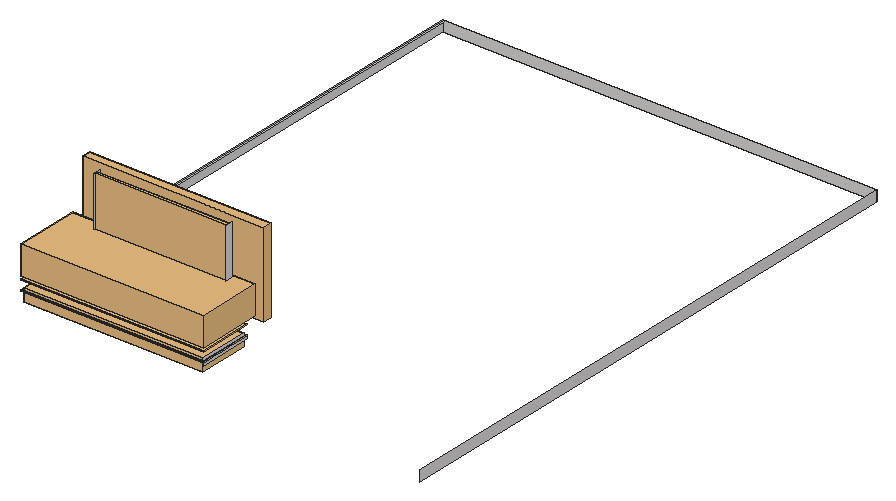
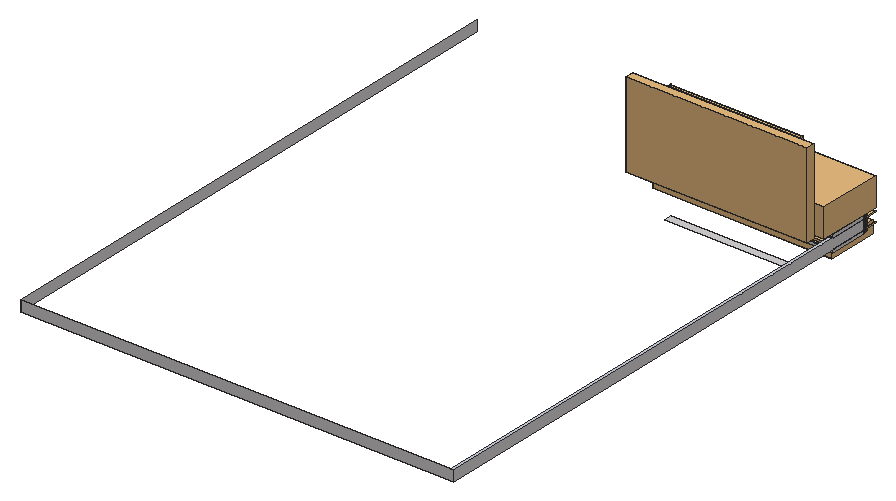
# SketchUp Ruby script. Lengths in inches.
U = 1.inch
M = Sketchup.active_model
def pt(a) = Geom::Point3d.new(a.map { |v| v * U })
def face(e, loops, mat)
  f = e.add_face(loops[0].map { |a| pt(a) })
  loops[1..].each { |l| e.add_face(l.map { |a| pt(a) }).erase! }
  f.material = f.back_material = mat if mat
  f
end
# faces: each face lists its corners as indices into pts; further lists are holes
def faces(e, pts, list, mat = nil) = list.each { |f| face(e, (f[0].is_a?(Array) ? f : [f]).map { |l| l.map { |i| pts[i] } }, mat) }
# xy, xz, yz: faces in a plane at the given z, y or x. An outline is a flat list of corners, or four numbers for a rectangle; further outlines are holes
def ring(l) = l.size == 4 ? [[l[0], l[1]], [l[2], l[1]], [l[2], l[3]], [l[0], l[3]]] : l.each_slice(2).to_a
def flat(e, list, mat, &to3) = list.each { |f| face(e, (f[0].is_a?(Array) ? f : [f]).map { |l| ring(l).map { |u, v| to3.(u, v) } }, mat) }
def xy(e, z, list, mat = nil) = flat(e, list, mat) { |x, y| [x, y, z] }
def xz(e, y, list, mat = nil) = flat(e, list, mat) { |x, z| [x, y, z] }
def yz(e, x, list, mat = nil) = flat(e, list, mat) { |y, z| [x, y, z] }
def lines(e, pts, list) = list.each { |a, b| e.add_line(pt(pts[a]), pt(pts[b])) }
# prism: a flat outline (further loops are holes) pulled along v
def prism(e, loops, v, mat = nil)
  f = face(e, loops, mat); d = Geom::Vector3d.new(v.map { |x| x * U })
  f.pushpull(f.normal.samedirection?(d) ? d.length : -d.length)
end
def box(e, o, s, mat = nil) = prism(e, [[o, [o[0] + s[0], o[1], o[2]], [o[0] + s[0], o[1] + s[1], o[2]], [o[0], o[1] + s[1], o[2]]]], [0, 0, s[2]], mat)
def at(x, y, z, deg = 0) = Geom::Transformation.translation(pt([x, y, z])) * Geom::Transformation.rotation(ORIGIN, Z_AXIS, deg.degrees)
def axes(o, x, y, z) = Geom::Transformation.new([*x, 0, *y, 0, *z, 0, *pt(o).to_a, 1])
def part(name) = M.definitions.add(name)
# library, detail: a bought-in or finely detailed component or shape, given as its bounding box
def library(name, o, s) = part(name).tap { |d| box(d.entities, o, s) }
def detail(e, o, s) = box(e.add_group.entities, o, s)
def put(e, d, t, mat = nil) = e.add_instance(d, t).tap { |i| i.material = mat if mat }
def group(e, t, mat = nil) = e.add_group.tap { |g| g.transformation = t; g.material = mat if mat }.entities
root = M.entities
M.materials.add("Outer Light - 1").color = [251, 216, 141]
M.materials.add("T METAL").color = [42, 41, 39]
M.materials.add("[Marble Carrara Floor Tile]").color = [204, 208, 219]
M.materials.add("[Quartz Light Brown]").color = [215, 212, 212]
c1 = library("Group\#43",[-0.5,-0.5,0],[204,61,1])
c2 = library("Group\#47",[0,0,-15.9],[195,66,15.9])
c3 = library("Group\#42",[-0.5,-0.5,0],[204,61,1])
c4 = library("Group\#21",[0,0,0],[201,72,32])
c5 = library("Glass Door Sliding Door 4 Panel on 2 Tracks _ Model by Pooh",[0,0,0],[157.59,4.01,102.67])
c6 = library("Garniza_zaclona",[1.52,0,0],[127.96,8.15,78.72])
xy(root,216,[[33,266,180,275]],"[Quartz Light Brown]")
xy(root,257.9,[[33,266,180,275]],"[Quartz Light Brown]")
xy(root,258,[[0,266,3,794]],"[Marble Carrara Floor Tile]")
xz(root,264,[[2,243,202,249]],"[Quartz Light Brown]")
xz(root,266,[[0,243,204,246],[0,246,0.5,247],[0,257,0.5,258],[0,258,3,261]],"[Quartz Light Brown]")
xz(root,794,[[0,246,483,258]],"[Quartz Light Brown]")
yz(root,0,[[222.76,243,223,246],[223,243,266,246],[266,246,266,247,223,247,223,257,266,257,266,258,794,258,794,246],[222.76,247,223,257],[222.76,258,223,261],
  [223,258,266,261]],"[Quartz Light Brown]")
yz(root,0.01,[[222.29,243,222.53,246],[222.29,247,222.53,257],[222.29,258,222.53,261]],"[Quartz Light Brown]")
yz(root,0.5,[[222.77,246,223,247],[223,246,266,247],[222.77,257,223,258],[223,257,266,258]],"[Quartz Light Brown]")
yz(root,0.51,[[222.3125,246,222.54,247],[222.3125,257,222.54,258]],"[Quartz Light Brown]")
yz(root,2,[[222.79,243,223,249],[223,243,264,249]],"[Quartz Light Brown]")
yz(root,2.01,[[222.37,243,222.58,249]],"[Quartz Light Brown]")
yz(root,3,[[222.8,258,223,261],[223,258,266,261]],"[Quartz Light Brown]")
yz(root,3.01,[[222.41,258,222.61,261]],"[Quartz Light Brown]")
yz(root,33,[[266,257.9,275,348]],"[Quartz Light Brown]")
yz(root,180,[[266,257.9,275,348]],"[Quartz Light Brown]")
yz(root,202,[[207,243,264,249]],"[Quartz Light Brown]")
yz(root,204,[[205,243,266,246]],"[Quartz Light Brown]")
yz(root,483,[[158,246,794,258]],"[Quartz Light Brown]")
p = [[1.2,216.55,246],[1.2,216.55,243],[1.28,216.33,243],[1.28,216.33,246],[3.38,216.49,249],[3.47,216.3,249],
  [3.47,216.3,243],[3.38,216.49,243],[1.11,216.77,246],[1.11,216.77,243],[3.3,216.68,249],[3.3,216.68,243],
  [3.22,216.88,249],[3.22,216.88,243],[1.03,216.99,246],[1.03,216.99,243],[3.14,217.07,249],[3.14,217.07,243],
  [0.96,217.21,246],[0.96,217.21,243],[3.0625,217.27,249],[3.0625,217.27,243],[0.88,217.4375,246],[0.88,217.4375,243],
  [2.99,217.46,249],[2.99,217.46,243],[0.81,217.66,246],[0.81,217.66,243],[2.92,217.66,249],[2.92,217.66,243],
  [0.74,217.89,246],[0.74,217.89,243],[2.85,217.86,249],[2.85,217.86,243],[0.68,218.11,246],[0.68,218.11,243],
  [2.78,218.06,249],[2.78,218.06,243],[0.61,218.34,246],[0.61,218.34,243],[2.72,218.26,249],[2.72,218.26,243],
  [0.55,218.57,246],[0.55,218.57,243],[2.66,218.46,249],[2.66,218.46,243],[2.6,218.66,249],[2.6,218.66,243],
  [0.5,218.8,246],[0.5,218.8,243],[2.55,218.86,249],[2.55,218.86,243],[0.44,219.03,246],[0.44,219.03,243],
  [2.49,219.0625,249],[2.49,219.0625,243],[0.39,219.26,246],[0.39,219.26,243],[2.44,219.26,249],[2.44,219.26,243],
  [0.35,219.49,246],[0.35,219.49,243],[2.39,219.47,249],[2.39,219.47,243],[0.3,219.72,246],[0.3,219.72,243],
  [2.35,219.67,249],[2.35,219.67,243],[0.26,219.95,246],[0.26,219.95,243],[2.31,219.88,249],[2.31,219.88,243],
  [2.27,220.08,249],[2.27,220.08,243],[0.22,220.18,246],[0.22,220.18,243],[2.23,220.29,249],[2.23,220.29,243],
  [0.1875,220.42,246],[0.1875,220.42,243],[2.2,220.5,249],[2.2,220.5,243],[0.15,220.65,246],[0.15,220.65,243],
  [2.17,220.7,249],[2.17,220.7,243],[0.125,220.88,246],[0.125,220.88,243],[2.14,220.91,249],[2.14,220.91,243],
  [0.1,221.12,246],[0.1,221.12,243],[2.11,221.12,249],[2.11,221.12,243],[0.08,221.35,246],[0.08,221.35,243],
  [2.09,221.33,249],[2.09,221.33,243],[2.07,221.54,249],[2.07,221.54,243],[0.06,221.59,246],[0.06,221.59,243],
  [2.05,221.74,249],[2.05,221.74,243],[0.04,221.82,246],[0.04,221.82,243],[2.03,221.95,249],[2.03,221.95,243],
  [0.02,222.06,246],[0.02,222.06,243],[2.02,222.16,249],[2.02,222.16,243],[0.01,222.29,246],[0.01,222.29,243],
  [2.01,222.37,249],[2.01,222.37,243],[0,222.76,246],[0,222.76,243],[0.01,222.53,243],[0.01,222.53,246],
  [2,222.79,249],[2.01,222.58,249],[2.01,222.58,243],[2,222.79,243],[1.75,216.52,247],[1.75,216.52,246],
  [1.83,216.3,246],[1.83,216.3,247],[1.66,216.73,247],[1.66,216.73,246],[1.58,216.94,247],[1.58,216.94,246],
  [1.5,217.16,247],[1.5,217.16,246],[1.43,217.375,247],[1.43,217.375,246],[1.36,217.59,247],[1.36,217.59,246],
  [1.29,217.8125,247],[1.29,217.8125,246],[1.22,218.03,247],[1.22,218.03,246],[1.16,218.25,247],[1.16,218.25,246],
  [1.1,218.47,247],[1.1,218.47,246],[1.04,218.69,247],[1.04,218.69,246],[0.98,218.91,247],[0.98,218.91,246],
  [0.93,219.14,247],[0.93,219.14,246],[0.88,219.36,247],[0.88,219.36,246],[0.84,219.59,247],[0.84,219.59,246],
  [0.79,219.8125,247],[0.79,219.8125,246],[0.75,220.04,247],[0.75,220.04,246],[0.72,220.26,247],[0.72,220.26,246],
  [0.68,220.49,247],[0.68,220.49,246],[0.65,220.72,247],[0.65,220.72,246],[0.62,220.94,247],[0.62,220.94,246],
  [0.6,221.17,247],[0.6,221.17,246],[0.57,221.4,247],[0.57,221.4,246],[0.55,221.625,247],[0.55,221.625,246],
  [0.54,221.86,247],[0.54,221.86,246],[0.52,222.08,247],[0.52,222.08,246],[0.51,222.3125,247],[0.51,222.3125,246],
  [0.5,222.77,247],[0.5,222.77,246],[0.51,222.54,246],[0.51,222.54,247],[1.2,216.55,257],[1.2,216.55,247],
  [1.28,216.33,247],[1.28,216.33,257],[1.11,216.77,257],[1.11,216.77,247],[1.03,216.99,257],[1.03,216.99,247],
  [0.96,217.21,257],[0.96,217.21,247],[0.88,217.4375,257],[0.88,217.4375,247],[0.81,217.66,257],[0.81,217.66,247],
  [0.74,217.89,257],[0.74,217.89,247],[0.68,218.11,257],[0.68,218.11,247],[0.61,218.34,257],[0.61,218.34,247],
  [0.55,218.57,257],[0.55,218.57,247],[0.5,218.8,257],[0.5,218.8,247],[0.44,219.03,257],[0.44,219.03,247],
  [0.39,219.26,257],[0.39,219.26,247],[0.35,219.49,257],[0.35,219.49,247],[0.3,219.72,257],[0.3,219.72,247],
  [0.26,219.95,257],[0.26,219.95,247],[0.22,220.18,257],[0.22,220.18,247],[0.1875,220.42,257],[0.1875,220.42,247],
  [0.15,220.65,257],[0.15,220.65,247],[0.125,220.88,257],[0.125,220.88,247],[0.1,221.12,257],[0.1,221.12,247],
  [0.08,221.35,257],[0.08,221.35,247],[0.06,221.59,257],[0.06,221.59,247],[0.04,221.82,257],[0.04,221.82,247],
  [0.02,222.06,257],[0.02,222.06,247],[0.01,222.29,257],[0.01,222.29,247],[0,222.76,257],[0,222.76,247],
  [0.01,222.53,247],[0.01,222.53,257],[1.75,216.52,258],[1.75,216.52,257],[1.83,216.3,257],[1.83,216.3,258],
  [1.66,216.73,258],[1.66,216.73,257],[1.58,216.94,258],[1.58,216.94,257],[1.5,217.16,258],[1.5,217.16,257],
  [1.43,217.375,258],[1.43,217.375,257],[1.36,217.59,258],[1.36,217.59,257],[1.29,217.8125,258],[1.29,217.8125,257],
  [1.22,218.03,258],[1.22,218.03,257],[1.16,218.25,258],[1.16,218.25,257],[1.1,218.47,258],[1.1,218.47,257],
  [1.04,218.69,258],[1.04,218.69,257],[0.98,218.91,258],[0.98,218.91,257],[0.93,219.14,258],[0.93,219.14,257],
  [0.88,219.36,258],[0.88,219.36,257],[0.84,219.59,258],[0.84,219.59,257],[0.79,219.8125,258],[0.79,219.8125,257],
  [0.75,220.04,258],[0.75,220.04,257],[0.72,220.26,258],[0.72,220.26,257],[0.68,220.49,258],[0.68,220.49,257],
  [0.65,220.72,258],[0.65,220.72,257],[0.62,220.94,258],[0.62,220.94,257],[0.6,221.17,258],[0.6,221.17,257],
  [0.57,221.4,258],[0.57,221.4,257],[0.55,221.625,258],[0.55,221.625,257],[0.54,221.86,258],[0.54,221.86,257],
  [0.52,222.08,258],[0.52,222.08,257],[0.51,222.3125,258],[0.51,222.3125,257],[0.5,222.77,258],[0.5,222.77,257],
  [0.51,222.54,257],[0.51,222.54,258],[4.63,216.19,258],[4.55,216.37,258],[4.55,216.37,261],[4.63,216.19,261],
  [1.28,216.33,258],[1.28,216.33,261],[1.2,216.55,261],[1.2,216.55,258],[4.46,216.54,258],[4.46,216.54,261],
  [1.11,216.77,261],[1.11,216.77,258],[4.38,216.72,258],[4.38,216.72,261],[4.3,216.9,258],[4.3,216.9,261],
  [1.03,216.99,261],[1.03,216.99,258],[4.22,217.08,258],[4.22,217.08,261],[0.96,217.21,261],[0.96,217.21,258],
  [4.14,217.26,258],[4.14,217.26,261],[0.88,217.4375,261],[0.88,217.4375,258],[4.07,217.44,258],[4.07,217.44,261],
  [0.81,217.66,261],[0.81,217.66,258],[4,217.625,258],[4,217.625,261],[3.93,217.81,258],[3.93,217.81,261],
  [0.74,217.89,261],[0.74,217.89,258],[3.86,217.99,258],[3.86,217.99,261],[0.68,218.11,261],[0.68,218.11,258],
  [3.8,218.18,258],[3.8,218.18,261],[0.61,218.34,261],[0.61,218.34,258],[3.73,218.36,258],[3.73,218.36,261],
  [0.55,218.57,261],[0.55,218.57,258],[3.67,218.55,258],[3.67,218.55,261],[0.5,218.8,261],[0.5,218.8,258],
  [3.62,218.74,258],[3.62,218.74,261],[3.5625,218.93,258],[3.5625,218.93,261],[0.44,219.03,261],[0.44,219.03,258],
  [3.51,219.12,258],[3.51,219.12,261],[0.39,219.26,261],[0.39,219.26,258],[3.46,219.31,258],[3.46,219.31,261],
  [0.35,219.49,261],[0.35,219.49,258],[3.41,219.5,258],[3.41,219.5,261],[0.3,219.72,261],[0.3,219.72,258],
  [3.37,219.69,258],[3.37,219.69,261],[0.26,219.95,261],[0.26,219.95,258],[3.33,219.88,258],[3.33,219.88,261],
  [3.29,220.07,258],[3.29,220.07,261],[0.22,220.18,261],[0.22,220.18,258],[3.25,220.27,258],[3.25,220.27,261],
  [0.1875,220.42,261],[0.1875,220.42,258],[3.22,220.46,258],[3.22,220.46,261],[0.15,220.65,261],[0.15,220.65,258],
  [3.18,220.65,258],[3.18,220.65,261],[0.125,220.88,261],[0.125,220.88,258],[3.16,220.85,258],[3.16,220.85,261],
  [3.13,221.04,258],[3.13,221.04,261],[0.1,221.12,261],[0.1,221.12,258],[3.1,221.24,258],[3.1,221.24,261],
  [0.08,221.35,261],[0.08,221.35,258],[3.08,221.43,258],[3.08,221.43,261],[0.06,221.59,261],[0.06,221.59,258],
  [3.0625,221.63,258],[3.0625,221.63,261],[0.04,221.82,261],[0.04,221.82,258],[3.05,221.82,258],[3.05,221.82,261],
  [0.02,222.06,261],[0.02,222.06,258],[3.03,222.02,258],[3.03,222.02,261],[3.02,222.21,258],[3.02,222.21,261],
  [0.01,222.29,261],[0.01,222.29,258],[3.01,222.41,258],[3.01,222.41,261],[0.01,222.53,258],[0.01,222.53,261],
  [0,222.76,261],[0,222.76,258],[3.01,222.61,258],[3,222.8,258],[3,222.8,261],[3.01,222.61,261]]
faces(root,p,[[0,1,2,3],[4,5,6,7],[8,9,1,0],[10,4,7,11],[12,10,11,13],[14,15,9,8],[16,12,13,17],[18,19,15,14],
  [20,16,17,21],[22,23,19,18],[24,20,21,25],[26,27,23,22],[28,24,25,29],[30,31,27,26],[32,28,29,33],[34,35,31,30],
  [36,32,33,37],[38,39,35,34],[40,36,37,41],[42,43,39,38],[44,40,41,45],[46,44,45,47],[48,49,43,42],[50,46,47,51],
  [52,53,49,48],[54,50,51,55],[56,57,53,52],[58,54,55,59],[60,61,57,56],[62,58,59,63],[64,65,61,60],[66,62,63,67],
  [68,69,65,64],[70,66,67,71],[72,70,71,73],[74,75,69,68],[76,72,73,77],[78,79,75,74],[80,76,77,81],[82,83,79,78],
  [84,80,81,85],[86,87,83,82],[88,84,85,89],[90,91,87,86],[92,88,89,93],[94,95,91,90],[96,92,93,97],[98,96,97,99],
  [100,101,95,94],[102,98,99,103],[104,105,101,100],[106,102,103,107],[108,109,105,104],[110,106,107,111],[112,113,109,108],[114,110,111,115],
  [116,117,118,119],[120,121,122,123],[124,125,126,127],[128,129,125,124],[130,131,129,128],[132,133,131,130],[134,135,133,132],[136,137,135,134],
  [138,139,137,136],[140,141,139,138],[142,143,141,140],[144,145,143,142],[146,147,145,144],[148,149,147,146],[150,151,149,148],[152,153,151,150],
  [154,155,153,152],[156,157,155,154],[158,159,157,156],[160,161,159,158],[162,163,161,160],[164,165,163,162],[166,167,165,164],[168,169,167,166],
  [170,171,169,168],[172,173,171,170],[174,175,173,172],[176,177,175,174],[178,179,177,176],[180,181,182,183],[184,185,186,187],[188,189,185,184],
  [190,191,189,188],[192,193,191,190],[194,195,193,192],[196,197,195,194],[198,199,197,196],[200,201,199,198],[202,203,201,200],[204,205,203,202],
  [206,207,205,204],[208,209,207,206],[210,211,209,208],[212,213,211,210],[214,215,213,212],[216,217,215,214],[218,219,217,216],[220,221,219,218],
  [222,223,221,220],[224,225,223,222],[226,227,225,224],[228,229,227,226],[230,231,229,228],[232,233,231,230],[234,235,233,232],[236,237,235,234],
  [238,239,240,241],[242,243,244,245],[246,247,243,242],[248,249,247,246],[250,251,249,248],[252,253,251,250],[254,255,253,252],[256,257,255,254],
  [258,259,257,256],[260,261,259,258],[262,263,261,260],[264,265,263,262],[266,267,265,264],[268,269,267,266],[270,271,269,268],[272,273,271,270],
  [274,275,273,272],[276,277,275,274],[278,279,277,276],[280,281,279,278],[282,283,281,280],[284,285,283,282],[286,287,285,284],[288,289,287,286],
  [290,291,289,288],[292,293,291,290],[294,295,293,292],[296,297,295,294],[298,299,300,301],[302,303,304,305],[306,307,308,309],[303,310,311,304],
  [309,308,312,313],[310,314,315,311],[314,316,317,315],[313,312,318,319],[316,320,321,317],[319,318,322,323],[320,324,325,321],[323,322,326,327],
  [324,328,329,325],[327,326,330,331],[328,332,333,329],[332,334,335,333],[331,330,336,337],[334,338,339,335],[337,336,340,341],[338,342,343,339],
  [341,340,344,345],[342,346,347,343],[345,344,348,349],[346,350,351,347],[349,348,352,353],[350,354,355,351],[354,356,357,355],[353,352,358,359],
  [356,360,361,357],[359,358,362,363],[360,364,365,361],[363,362,366,367],[364,368,369,365],[367,366,370,371],[368,372,373,369],[371,370,374,375],
  [372,376,377,373],[376,378,379,377],[375,374,380,381],[378,382,383,379],[381,380,384,385],[382,386,387,383],[385,384,388,389],[386,390,391,387],
  [389,388,392,393],[390,394,395,391],[394,396,397,395],[393,392,398,399],[396,400,401,397],[399,398,402,403],[400,404,405,401],[403,402,406,407],
  [404,408,409,405],[407,406,410,411],[408,412,413,409],[411,410,414,415],[412,416,417,413],[416,418,419,417],[415,414,420,421],[418,422,423,419],
  [424,425,426,427],[428,429,430,431]],"[Quartz Light Brown]")
put(root,c1,at(0.5,205.5,257),"Outer Light - 1")
put(root,c2,axes([2,207,249],[1.02564,0,0],[0,0.86364,0],[0,0,0.85]),"[Quartz Light Brown]")
put(root,c3,at(0.5,205.5,246),"Outer Light - 1")
put(root,c4,axes([0.25,205.25,261],[1.01368,0,0],[0,1,0],[0,0,1]),"T METAL")
put(root,c5,axes([33,267,258],[0.93279,0,0],[0,1,0],[0,0,0.87661]),"[Quartz Light Brown]")
put(root,c6,axes([9,277.55,258],[1.58151,0,0],[0,1.1771,0],[0,0,1.20432]))
